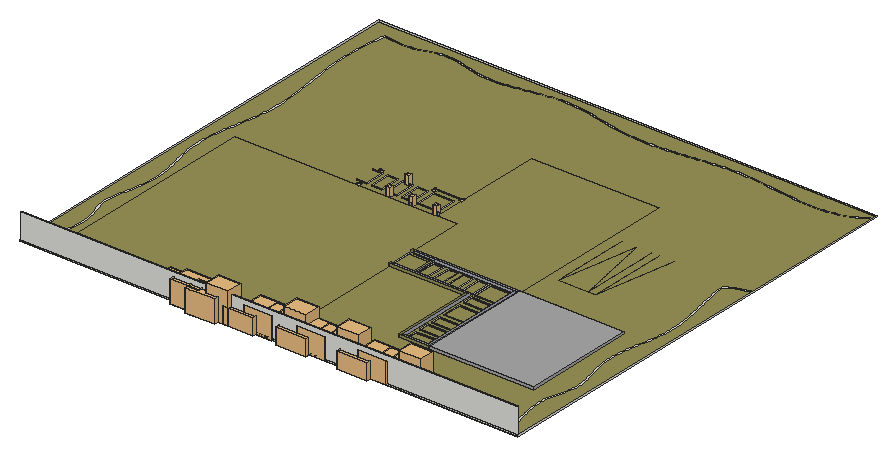
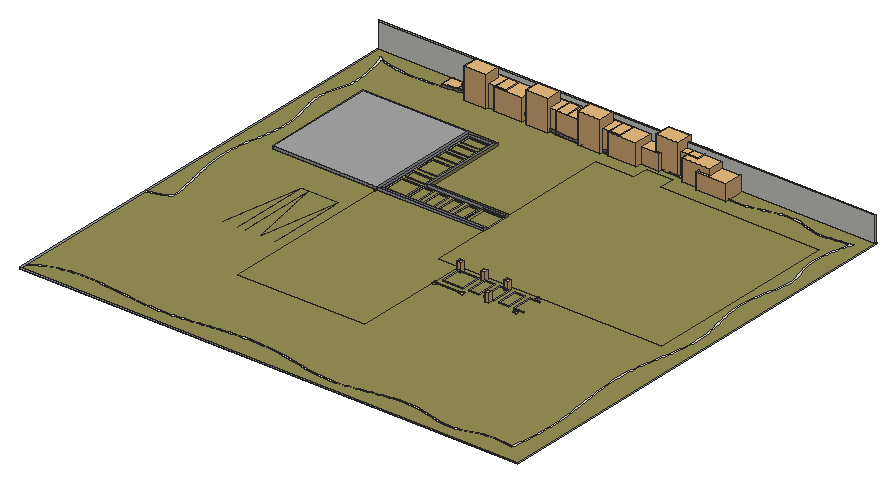
# SketchUp Ruby script. Lengths in inches.
U = 1.inch
M = Sketchup.active_model
def pt(a) = Geom::Point3d.new(a.map { |v| v * U })
def face(e, loops, mat)
  f = e.add_face(loops[0].map { |a| pt(a) })
  loops[1..].each { |l| e.add_face(l.map { |a| pt(a) }).erase! }
  f.material = f.back_material = mat if mat
  f
end
# faces: each face lists its corners as indices into pts; further lists are holes
def faces(e, pts, list, mat = nil) = list.each { |f| face(e, (f[0].is_a?(Array) ? f : [f]).map { |l| l.map { |i| pts[i] } }, mat) }
# xy, xz, yz: faces in a plane at the given z, y or x. An outline is a flat list of corners, or four numbers for a rectangle; further outlines are holes
def ring(l) = l.size == 4 ? [[l[0], l[1]], [l[2], l[1]], [l[2], l[3]], [l[0], l[3]]] : l.each_slice(2).to_a
def flat(e, list, mat, &to3) = list.each { |f| face(e, (f[0].is_a?(Array) ? f : [f]).map { |l| ring(l).map { |u, v| to3.(u, v) } }, mat) }
def xy(e, z, list, mat = nil) = flat(e, list, mat) { |x, y| [x, y, z] }
def xz(e, y, list, mat = nil) = flat(e, list, mat) { |x, z| [x, y, z] }
def yz(e, x, list, mat = nil) = flat(e, list, mat) { |y, z| [x, y, z] }
def lines(e, pts, list) = list.each { |a, b| e.add_line(pt(pts[a]), pt(pts[b])) }
# prism: a flat outline (further loops are holes) pulled along v
def prism(e, loops, v, mat = nil)
  f = face(e, loops, mat); d = Geom::Vector3d.new(v.map { |x| x * U })
  f.pushpull(f.normal.samedirection?(d) ? d.length : -d.length)
end
def box(e, o, s, mat = nil) = prism(e, [[o, [o[0] + s[0], o[1], o[2]], [o[0] + s[0], o[1] + s[1], o[2]], [o[0], o[1] + s[1], o[2]]]], [0, 0, s[2]], mat)
def at(x, y, z, deg = 0) = Geom::Transformation.translation(pt([x, y, z])) * Geom::Transformation.rotation(ORIGIN, Z_AXIS, deg.degrees)
def axes(o, x, y, z) = Geom::Transformation.new([*x, 0, *y, 0, *z, 0, *pt(o).to_a, 1])
def part(name) = M.definitions.add(name)
# library, detail: a bought-in or finely detailed component or shape, given as its bounding box
def library(name, o, s) = part(name).tap { |d| box(d.entities, o, s) }
def detail(e, o, s) = box(e.add_group.entities, o, s)
def put(e, d, t, mat = nil) = e.add_instance(d, t).tap { |i| i.material = mat if mat }
def group(e, t, mat = nil) = e.add_group.tap { |g| g.transformation = t; g.material = mat if mat }.entities
root = M.entities
M.materials.add("M03_Pewter_Shine").color = [168, 168, 168]
M.materials.add("Marble_01_1K").color = [230, 221, 211]
M.materials.add("Marble_20_1K").color = [172, 173, 182]
M.materials.add("Material__4").color = [36, 36, 36]
M.materials.add("Material__6").color = [79, 108, 5]
M.materials.add("Plaster_06_1K").color = [141, 135, 122]
M.materials.add("Soil_04_1K").color = [152, 146, 88]
M.materials.add("calathea lutea").color = [121, 145, 80]
c1 = library("light",[-4,-4,0],[8,8,0.01])
c2 = library("tt",[-12.4,-12.1,0],[24.8,24.2,0.01])
c3 = library("ew",[-14.92,-16.84,0],[29.84,33.68,0.01])
c4 = part("Group\#156")
g1 = group(c4.entities,at(8.61,38.85,0))
xy(g1,0,[[0,0,2.82,19.1,22.58,0],[22.58,0,2.82,19.1,22.58,19.1]],"calathea lutea")
p = [[2.82,19.1,0],[7.19,48.22,5.13],[10.77,48.22,5.13],[12.74,48.22,5.13],[22.58,48.22,5.13],[22.58,19.1,0]]
faces(g1,p,[[0,1,2,3,4,5]],"calathea lutea")
g2 = group(c4.entities,at(-0.77,-7.77,0))
p = [[14.8125,23.31,1.46],[21.35,23.31,0],[14.8125,0,1.46],[21.35,0,0],[27.89,0,1.46],[27.89,23.31,1.46],
  [8.27,46.62,2.92],[21.35,46.62,0],[34.4375,46.62,2.92],[4.47,23.31,6.43],[0,0,8.59],[33.76,0,4.28],
  [33.76,23.31,4.28]]
faces(g2,p,[[0,1,2],[3,2,1],[4,3,5],[1,5,3],[6,7,0],[1,0,7],[5,1,8],[7,8,1],
  [9,0,2,10],[11,4,5,12],[9,6,0],[12,5,8]],"calathea lutea")
c5 = part("Group\#150")
xy(c5.entities,0,[[0,0,0,33.87,27.21,33.87,19.71,0]],"calathea lutea")
c6 = part("Group\#157")
xy(c6.entities,1.04,[[21.13,33.87,21.13,57.59,32.375,57.59,27.12,33.87]],"calathea lutea")
xy(c6.entities,1.32,[[0.12,33.87,7.74,57.59]],"calathea lutea")
p = [[7.74,33.87,1.32],[11.8,57.59,0.61],[15.24,57.59,0],[15.24,33.87,0],[18.43,57.59,0.5625],[21.13,57.59,1.04],
  [21.13,33.87,1.04],[15.24,77.7,2.36],[21.13,77.7,3.4],[7.74,57.59,1.32],[7.74,77.7,3.69],[36.83,77.7,3.4],
  [32.375,57.59,1.04],[0.12,57.59,1.32],[0.12,77.7,3.69]]
faces(c6.entities,p,[[0,1,2,3],[3,2,4],[3,4,5,6],[7,2,1],[8,4,2,7],[0,9,1],[7,1,9,10],[8,5,4],
  [11,12,5,8],[10,9,13,14]],"calathea lutea")
put(c6.entities,c5,axes([0,-16.9375,0],[1,0,0],[0,1.5,0],[0,0,1]))
c7 = part("Group\#155")
g3 = group(c7.entities,at(0,-17.3,0))
xy(g3,0,[[0,0,28.07,51.9]],"calathea lutea")
g4 = group(c7.entities,at(0.9,34.6,0))
xy(g4,0,[[13.14,0,13.14,26.22,16.85,26.22],[13.14,0,16.85,26.22,20.16,26.22,20.16,0]],"calathea lutea")
p = [[6.36,0,1.82],[9.95,26.22,0.86],[13.14,26.22,0],[13.14,0,0],[20.16,0,0],[20.16,26.22,0],
  [27.07,26.22,1.22],[27.07,0,1.22],[13.14,49.5625,5.91],[20.16,49.5625,5.91],[16.85,26.22,0],[27.07,49.5625,7.125],
  [6.36,26.22,1.82],[6.36,49.5625,7.72],[0,0,4.78],[0,26.22,4.78],[0,49.5625,10.6875]]
faces(g4,p,[[0,1,2,3],[4,5,6,7],[8,2,1],[9,10,2,8],[9,5,10],[11,6,5,9],[0,12,1],[8,1,12,13],
  [14,15,12,0],[13,12,15,16]],"calathea lutea")
c8 = part("Group\#154")
put(c8.entities,c5,axes([0,-16.9375,0],[1,0,0],[0,1.5,0],[0,0,1]))
g5 = group(c8.entities,at(-0.23,33.4,-0.35))
p = [[15.12,39.14,-19.87],[15.12,20.54,-11.86],[11.68,20.84,-11.33],[21.02,39.66,-18.97],[18.3125,20.82,-11.37],[7.62,21.2,-10.71],
  [7.62,39.8,-18.72],[21.02,21.06,-10.96],[36.72,39.66,-18.97],[32.26,21.06,-10.96],[0,21.2,-10.71],[0,39.8,-18.72],
  [7.62,0.66,1.15],[15.12,0,0],[21.02,0.52,0.9],[27.01,0.52,0.9],[0,0.66,1.15]]
faces(g5,p,[[0,1,2],[3,4,1,0],[0,2,5,6],[3,7,4],[8,9,7,3],[6,5,10,11],[12,2,1,13],[13,1,4],
  [13,4,7,14],[12,5,2],[14,7,9,15],[16,10,5,12]],"calathea lutea")
c9 = part("Foliage cluster")
put(c9.entities,c4,axes([37.24,8.07,75.17],[1,0,0],[0,0.45554,-0.89021],[0,0.89021,0.45554]))
put(c9.entities,c6,axes([69.44,65.48,16.68],[-0.53288,-0.84619,0],[0.14694,-0.09253,0.98481],[-0.83334,0.52478,0.17365]))
put(c9.entities,c7,axes([47.9375,70.43,17.04],[0.74664,-0.66523,0],[0.11552,0.12965,0.98481],[-0.65512,-0.7353,0.17365]))
put(c9.entities,c4,axes([76.19,10.66,75.17],[0.70711,0.70711,0],[-0.32212,0.32212,-0.89021],[-0.62948,0.62948,0.45554]))
put(c9.entities,c4,axes([101.91,40.03,75.17],[0,1,0],[-0.45554,0,-0.89021],[-0.89021,0,0.45554]))
put(c9.entities,c4,axes([99.32,78.99,75.17],[-0.70711,0.70711,0],[-0.32212,-0.32212,-0.89021],[-0.62948,-0.62948,0.45554]))
put(c9.entities,c7,axes([34.81,63.36,17.04],[0.99956,-0.02967,0],[0.00515,0.17357,0.98481],[-0.02922,-0.98437,0.17365]))
put(c9.entities,c7,axes([48,37.4,15.8],[-0.14436,0.98953,0],[-0.40248,-0.05871,0.91355],[0.90398,0.13188,0.40674]))
put(c9.entities,c6,axes([56.87,39.77,12.28],[-0.67695,0.4263,0],[-0.18016,-0.28609,0.72505],[0.38636,0.61353,0.33809]))
put(c9.entities,c6,axes([36.12,43.25,12.28],[0.18947,0.77724,0],[-0.32848,0.08007,0.72505],[0.70442,-0.17172,0.33809]))
put(c9.entities,c8,axes([35.1,54.93,11.375],[0.79719,0.06694,0],[-0.03636,0.43302,0.6717],[0.05621,-0.66934,0.43454]))
put(c9.entities,c6,axes([41.66,47.32,12.28],[0.45082,0.66088,0],[-0.2793,0.19053,0.72505],[0.59896,-0.40858,0.33809]))
put(c9.entities,c6,axes([47.89,59.4,12.28],[0.79719,0.06694,0],[-0.02829,0.33691,0.72505],[0.06067,-0.7225,0.33809]))
put(c9.entities,c8,axes([29.53,49.96,11.375],[0.65692,0.45657,0],[-0.248,0.35682,0.6717],[0.38335,-0.55156,0.43454]))
put(c9.entities,c8,axes([29.9,49.27,12.86],[0.34062,0.72386,0],[-0.22849,0.10752,0.7591],[0.68685,-0.32321,0.25252]))
put(c9.entities,c8,axes([36.33,48.82,8.99],[0.09232,0.62522,0],[-0.3396,0.05015,0.53064],[0.52495,-0.07752,0.34329]))
put(c9.entities,c8,axes([49.82,38.52,8.99],[-0.54622,0.31791,0],[-0.17268,-0.29669,0.53064],[0.26692,0.45862,0.34329]))
put(c9.entities,c8,axes([55.68,39.21,8.99],[-0.632,0.00221,0],[-0.0012,-0.34328,0.53064],[0.00185,0.53064,0.34329]))
c10 = library("Group\#28",[0,0,0],[86.94,78.77,46.4375])
c11 = library("Group\#14",[-978.71,-103.24,719.12],[90.2,76.4,68.29])
c12 = library("Group\#13",[-906.16,-138.28,686.8],[98.25,106.18,75.79])
c13 = library("Group\#202",[-3.47,-2.45,12.47],[53.14,54.93,75.51])
c14 = library("Group\#54",[0,0,0],[2062.46,2062.46,4833.66])
c15 = part("Landscape+Light")
put(c15.entities,c14,at(-2096.57,-1031.23,-3775.98))
c16 = library("t1",[-17.79,-17.21,0],[35.58,34.42,0.01])
c17 = part("Group\#44")
put(c17.entities,c9,axes([161.54,105.34,6.01],[0.19523,-0.19694,0],[0.19694,0.19523,0],[0,0,0.24957]))
put(c17.entities,c10,axes([0,37.34,0.92],[0.83,0,0],[0,0.83,0],[0,0,0.83]))
put(c17.entities,c11,axes([859.63,139.86,-568.1],[0.79,0,0],[0,0.79,0],[0,0,0.79]),"Material__4")
put(c17.entities,c12,axes([669.69,145.1,-472.48],[0.69,0,0],[0,0.69,0],[0,0,0.69]),"Material__6")
put(c17.entities,c13,at(132.78,74.93,-12.6))
xy(root,0,[[480.859,22.514,469.576,22.663,458.203,23.333,446.764,24.525,435.279,26.15,423.754,28.103,412.194,30.286,400.608,32.597,389.002,34.937,377.385,37.206,365.763,39.306,354.147,41.14,342.544,42.61,330.964,43.618,319.414,44.07,307.903,43.869,296.431,42.924,284.954,41.245,273.478,39.01,262.023,36.415,250.609,33.658,239.255,30.938,227.977,28.456,216.79,26.418,205.705,25.031,194.737,24.507,183.905,25.065,173.26,26.904,162.899,29.804,152.679,33.204,142.425,36.559,131.969,39.345,121.109,41.119,109.806,41.864,98.284,41.752,86.773,40.964,75.503,39.681,64.7,38.09,54.587,36.377,45.348,34.713,36.369,33.075,37.514,35.489,38.66,37.904,39.808,40.342,41.005,43.315,42.25,47.021,43.529,51.453,44.835,56.612,46.164,62.502,47.513,69.13,48.883,76.509,50.312,84.622,51.732,93.308,53.035,102.439,54.109,111.884,54.846,121.51,55.138,131.183,54.879,140.766,53.965,150.125,52.298,159.138,49.937,167.888,47.159,176.49,44.27,185.043,41.586,193.648,39.4375,202.41,38.14,211.376,37.733,220.458,38.089,229.635,39.079,238.896,40.576,248.232,42.459,257.636,44.605,267.101,46.895,276.617,49.21,286.176,51.434,295.765,53.449,305.374,55.14,314.99,56.393,324.601,57.112,334.213,57.309,343.854,57.039,353.523,56.36,363.215,55.325,372.925,53.993,382.649,52.42,392.381,50.664,402.117,48.783,411.85,46.833,421.576,44.873,431.291,42.962,440.991,41.158,450.67,39.521,460.325,38.109,469.951,36.982,479.546,36.201,489.105,35.799,498.606,35.753,508.044,36.031,517.421,36.604,526.741,37.439,536.006,38.507,545.221,39.776,554.389,41.216,563.513,42.797,572.596,44.486,581.644,46.256,590.658,48.074,599.642,49.912,608.601,51.739,617.537,53.524,626.455,55.239,635.357,56.852,644.248,58.336,653.13,59.659,662.006,60.793,670.882,61.708,679.759,62.385,688.651,62.836,697.561,63.075,706.489,63.117,715.435,62.976,724.398,62.669,733.377,62.209,742.37,61.613,751.377,60.895,760.397,60.07,769.428,59.153,778.469,58.159,787.52,57.104,796.579,56.004,805.645,54.872,814.718,53.725,823.796,52.578,832.878,51.446,841.963,50.344,851.051,49.287,860.139,48.292,869.229,47.373,878.317,46.547,887.404,45.828,896.488,45.232,905.569,44.774,914.645,44.47,923.716,44.336,932.78,44.388,941.837,44.633,950.881,45.057,959.917,45.639,968.957,46.358,978.013,47.193,987.098,48.123,996.223,49.126,1005.402,50.183,1014.646,51.273,1023.969,52.374,1033.383,53.47,1042.887,63.941,1041.194,74.718,1039.586,85.979,1038.273,97.499,1037.444,109.045,1037.281,120.387,1037.965,131.296,1039.672,141.787,1042.409,152.064,1045.749,162.297,1049.166,172.66,1052.115,183.306,1054.029,194.148,1054.654,205.125,1054.182,216.221,1052.832,227.421,1050.819,238.712,1048.35,250.08,1045.633,261.509,1042.869,272.98,1040.258,284.474,1038.001,295.969,1036.292,307.458,1035.315,318.985,1035.087,330.551,1035.517,342.148,1036.509,353.768,1037.967,365.402,1039.794,377.041,1041.891,388.677,1044.16,400.301,1046.503,411.905,1048.82,423.483,1051.01,435.027,1052.972,446.531,1054.607,457.988,1055.811,469.38,1056.492,480.682,1056.65,491.897,1056.336,503.03,1055.604,514.087,1054.507,525.073,1053.098,535.995,1051.428,546.859,1049.551,557.67,1047.517,568.436,1045.38,579.161,1043.19,589.853,1040.999,600.516,1038.859,611.158,1036.82,621.784,1034.934,632.4,1033.251,643.011,1031.822,653.624,1030.696,664.256,1029.907,674.915,1029.439,685.6,1029.266,696.309,1029.363,707.041,1029.703,717.794,1030.262,728.567,1031.013,739.357,1031.931,750.162,1032.99,760.981,1034.164,771.812,1035.426,782.653,1036.752,793.503,1038.115,804.36,1039.488,815.221,1040.846,826.086,1042.163,836.953,1043.412,847.819,1044.567,858.684,1045.601,869.546,1046.488,880.403,1047.202,891.253,1047.716,902.095,1048.004,912.927,1048.038,923.744,1047.798,934.548,1047.297,945.358,1046.573,956.196,1045.662,967.083,1044.598,978.04,1043.418,989.088,1042.158,1000.249,1040.852,1011.544,1039.536,1022.995,1038.246,1034.624,1037.016,1046.425,1035.892,1058.357,1034.938,1070.374,1034.219,1082.429,1033.8,1094.476,1033.748,1106.468,1034.125,1118.359,1034.996,1130.102,1036.427,1141.651,1038.479,1152.963,1041.215,1163.991,1044.698,1174.694,1048.99,1185.032,1054.156,1194.964,1060.26,1204.463,1067.348,1204.463,1063.517,1194.306,1056.225,1183.681,1050.02,1172.637,1044.829,1161.225,1040.58,1149.495,1037.198,1137.499,1034.61,1125.287,1032.743,1112.909,1031.522,1100.417,1030.875,1087.86,1030.727,1075.29,1031.006,1062.757,1031.637,1050.312,1032.548,1038.005,1033.665,1025.886,1034.914,1013.972,1036.238,1002.24,1037.598,990.666,1038.954,979.229,1040.266,967.904,1041.497,956.667,1042.606,945.496,1043.554,934.367,1044.303,923.256,1044.8125,912.14,1045.045,901.005,1044.985,889.852,1044.659,878.682,1044.096,867.497,1043.324,856.3,1042.372,845.091,1041.27,833.874,1040.047,822.65,1038.731,811.42,1037.351,800.187,1035.937,788.953,1034.517,777.719,1033.12,766.488,1031.776,755.261,1030.513,744.04,1029.36,732.827,1028.347,721.624,1027.501,710.434,1026.854,699.257,1026.432,688.096,1026.265,676.953,1026.383,665.829,1026.814,654.726,1027.587,643.647,1028.724,632.585,1030.192,621.535,1031.934,610.49,1033.893,599.443,1036.013,588.388,1038.236,577.317,1040.506,566.224,1042.765,555.102,1044.958,543.944,1047.026,532.744,1048.913,521.494,1050.5625,510.189,1051.917,498.821,1052.92,487.384,1053.514,475.871,1053.643,464.275,1053.249,452.59,1052.287,440.82,1050.812,428.974,1048.933,417.061,1046.761,405.089,1044.407,393.068,1041.981,381.005,1039.594,368.911,1037.355,356.794,1035.377,344.663,1033.769,332.526,1032.642,320.393,1032.106,308.272,1032.272,296.173,1033.248,284.108,1035.019,272.098,1037.379,260.165,1040.104,248.328,1042.971,236.611,1045.755,225.033,1048.235,213.615,1050.185,202.379,1051.383,191.346,1051.605,180.537,1050.629,169.95,1048.319,159.451,1045.08,148.858,1041.508,137.986,1038.203,126.654,1035.76,114.824,1034.505,102.716,1034.276,90.578,1034.864,78.657,1036.056,67.199,1037.643,56.085,1039.364,54.849,1028.711,53.616,1018.189,52.414,1007.782,51.273,997.471,50.221,987.24,49.288,977.071,48.504,966.946,47.898,956.847,47.499,946.758,47.335,936.66,47.41,926.547,47.705,916.418,48.196,906.275,48.863,896.12,49.684,885.955,50.637,875.779,51.7,865.596,52.851,855.406,54.07,845.21,55.334,835.011,56.621,824.81,57.91,814.607,59.179,804.405,60.407,794.205,61.571,784.008,62.65,773.816,63.623,763.63,64.467,753.452,65.16,743.283,65.682,733.124,66.011,722.977,66.124,712.844,66,702.725,65.618,692.622,64.955,682.537,63.992,672.471,62.745,662.421,61.255,652.383,59.565,642.351,57.718,632.321,55.756,622.287,53.722,612.244,51.658,602.187,49.608,592.112,47.613,582.012,45.717,571.884,43.961,561.722,42.389,551.521,41.044,541.275,39.967,530.981,39.202,520.632,38.79,510.224,38.776,499.752,39.2,489.21,40.096,478.595,41.416,467.91,43.077,457.161,44.997,446.356,47.093,435.5,49.282,424.601,51.481,413.664,53.608,402.697,55.579,391.707,57.313,380.699,58.725,369.681,59.734,358.659,60.257,347.64,60.21,336.63,59.511,325.636,58.126,314.667,56.185,303.736,53.855,292.861,51.305,282.055,48.701,271.336,46.211,260.719,44.002,250.22,42.242,239.854,41.098,229.638,40.737,219.587,41.327,209.717,43.02,200.04,45.663,190.492,48.819,180.939,52.038,171.244,54.874,161.268,56.888,150.881,57.922,140.1,58.119,129.101,57.636,118.071,56.633,107.192,55.267,96.652,53.696,86.635,52.077,77.325,50.523,68.896,48.995,61.397,47.487,54.813,46.001,49.129,44.536,44.328,43.092,40.394,41.666,37.135,51.57,38.889,61.787,40.655,72.801,42.341,84.391,43.746,96.317,44.665,108.34,44.894,120.222,44.229,131.723,42.467,142.713,39.607,153.328,36.152,163.746,32.683,174.144,29.778,184.696,27.998,195.475,27.511,206.466,28.115,217.648,29.594,229,31.732,240.502,34.312,252.134,37.117,263.875,39.933,275.705,42.541,287.603,44.727,299.55,46.273,311.525,47.01,323.519,46.981,335.523,46.292,347.528,45.052,359.526,43.367,371.508,41.344,383.465,39.09,395.39,36.713,407.273,34.318,419.105,32.013,430.88,29.905,442.586,28.101,454.218,26.708,465.764,25.831,477.225,25.508,488.605,25.69,499.912,26.321,511.151,27.347,522.329,28.712,533.453,30.362,544.53,32.24,555.565,34.293,566.566,36.465,577.539,38.702,588.49,40.947,599.426,43.146,610.353,45.243,621.279,47.185,632.209,48.915,643.151,50.379,654.11,51.521,665.091,52.307,676.093,52.757,687.114,52.898,698.153,52.758,709.208,52.366,720.276,51.749,731.356,50.936,742.447,49.955,753.545,48.833,764.65,47.599,775.759,46.281,786.872,44.907,797.985,43.504,809.097,42.102,820.206,40.727,831.31,39.409,842.408,38.174,853.498,37.052,864.577,36.07,875.645,35.256,886.698,34.639,897.736,34.246,908.756,34.105,919.757,34.244,930.747,34.665,941.748,35.332,952.781,36.207,963.871,37.252,975.039,38.43,986.309,39.702,997.702,41.032,1009.243,42.38,1020.952,43.709,1032.854,44.981,1044.954,46.15,1057.211,47.15,1069.575,47.908,1081.999,48.353,1094.433,48.415,1106.827,48.023,1119.133,47.104,1131.302,45.588,1143.285,43.404,1155.033,40.481,1166.497,36.747,1177.627,32.131,1176.661,34.304,1175.695,36.527,1174.719,39.093,1173.734,42.055,1172.739,45.418,1171.734,49.186,1170.719,53.365,1169.695,57.96,1168.661,62.975,1167.617,68.415,1166.557,74.284,1165.459,80.555,1164.367,87.17,1163.328,94.072,1162.393,101.204,1161.61,108.508,1161.028,115.926,1160.696,123.401,1160.663,130.876,1160.979,138.293,1161.693,145.594,1162.854,152.722,1164.468,159.642,1166.419,166.384,1168.568,172.991,1170.775,179.506,1172.9,185.972,1174.806,192.43,1176.351,198.924,1177.405,205.495,1177.944,212.156,1178.02,218.902,1177.683,225.73,1176.987,232.633,1175.982,239.607,1174.722,246.647,1173.258,253.748,1171.641,260.906,1169.925,268.115,1168.162,275.37,1166.402,282.667,1164.699,290,1163.104,297.365,1161.669,304.757,1160.447,312.17,1159.489,319.601,1158.845,327.044,1158.519,334.496,1158.486,341.954,1158.72,349.418,1159.197,356.884,1159.889,364.351,1160.772,371.816,1161.82,379.278,1163.007,386.735,1164.306,394.184,1165.693,401.623,1167.142,409.051,1168.627,416.465,1170.122,423.863,1171.601,431.244,1173.039,438.604,1174.41,445.943,1175.689,453.258,1176.848,460.546,1177.864,467.806,1178.71,475.037,1179.36,482.234,1179.793,489.398,1180.012,496.53,1180.03,503.631,1179.862,510.703,1179.519,517.75,1179.016,524.773,1178.365,531.775,1177.58,538.758,1176.674,545.723,1175.661,552.674,1174.552,559.613,1173.363,566.542,1172.106,573.462,1170.794,580.377,1169.441,587.289,1168.059,594.2,1166.663,601.112,1165.264,608.027,1163.878,614.947,1162.516,621.876,1161.192,628.815,1159.92,635.766,1158.712,642.732,1157.581,649.715,1156.542,656.717,1155.607,663.741,1154.79,670.788,1154.104,677.862,1154.572,684.97,1160.145,692.147,1175.308,699.425,1204.463,706.821,1204.463,703.683,1176.673,696.07,1162.475,688.712,1157.456,681.529,1157.204,674.442,1157.945,667.378,1158.824,660.316,1159.828,653.253,1160.942,646.187,1162.151,639.118,1163.439,632.043,1164.792,624.96,1166.195,617.869,1167.634,610.766,1169.092,603.651,1170.555,596.522,1172.007,589.376,1173.433,582.212,1174.819,575.029,1176.148,567.823,1177.405,560.595,1178.576,553.341,1179.645,546.06,1180.596,538.751,1181.414,531.411,1182.084,524.038,1182.589,516.632,1182.914,509.189,1183.044,501.71,1182.963,494.191,1182.656,486.633,1182.108,479.036,1181.329,471.412,1180.347,463.768,1179.195,456.103,1177.901,448.421,1176.496,440.724,1175.009,433.013,1173.47,425.29,1171.908,417.557,1170.353,409.818,1168.835,402.073,1167.382,394.326,1166.023,386.58,1164.788,378.836,1163.705,371.097,1162.803,363.366,1162.11,355.645,1161.656,347.937,1161.469,340.244,1161.575,332.569,1162.005,324.913,1162.781,317.269,1163.879,309.619,1165.243,301.966,1166.816,294.318,1168.539,286.68,1170.354,279.059,1172.201,271.46,1174.022,263.888,1175.758,256.349,1177.347,248.847,1178.729,241.385,1179.842,233.968,1180.624,226.599,1181.012,219.283,1180.942,212.025,1180.346,204.83,1179.166,197.72,1177.455,190.748,1175.383,183.882,1173.117,177.07,1170.819,170.259,1168.646,163.4,1166.75,156.442,1165.28,149.333,1164.302,141.997,1163.772,134.471,1163.641,126.824,1163.855,119.127,1164.362,111.445,1165.106,103.848,1166.033,96.404,1167.089,89.177,1168.217,82.236,1169.362,75.643,1170.472,69.476,1171.556,63.797,1172.628,58.59,1173.687,53.849,1174.731,49.573,1175.76,45.758,1176.771,42.402,1177.76,39.506,1178.718,37.074,1179.638,35.072,1180.549,33.15,1181.461,31.229,1182.372,29.308,1183.284,27.387,1183.794,26.3125,1184.195,25.466,1173.842,30.55,1163.128,34.769,1152.093,38.186,1140.779,40.863,1129.231,42.863,1117.493,44.247,1105.612,45.08,1093.632,45.424,1081.602,45.344,1069.567,44.904,1057.573,44.168,1045.666,43.202,1033.892,42.071,1022.293,40.839,1010.869,39.548,999.6,38.234,988.463,36.932,977.4375,35.677,966.502,34.504,955.635,33.449,944.815,32.547,934.022,31.835,923.235,31.347,912.434,31.119,901.617,31.166,890.792,31.463,879.958,31.985,869.117,32.705,858.272,33.598,847.424,34.635,836.574,35.792,825.724,37.042,814.876,38.358,804.031,39.715,793.192,41.086,782.359,42.446,771.534,43.769,760.72,45.028,749.918,46.197,739.129,47.252,728.356,48.165,717.601,48.912,706.864,49.466,696.149,49.802,685.457,49.895,674.789,49.719,664.146,49.248,653.531,48.457,642.934,47.331,632.339,45.902,621.739,44.22,611.13,42.336,600.504,40.301,589.857,38.164,579.182,35.976,568.473,33.789,557.724,31.655,546.929,29.624,536.083,27.748,525.178,26.079,514.209,24.668,503.17,23.569,492.055,22.833],[811.725,356.108,859.725,356.125]])
xy(root,0,[[460.425,50.78,522.398,50.78,522.398,88.78,613.506,88.78,613.506,562.78,566.192,562.78,566.192,565.82,561.692,565.82,561.692,562.78,76.506,562.78,76.506,88.78,460.425,88.78],[[797.8125,154.932,797.8125,356.108,613.506,356.108,613.506,368.125,661.506,368.125,661.506,415.985,613.506,415.985,613.506,428.082,870.828,428.082,870.828,154.932],[803.8125,160.932,864.828,160.932,864.828,422.082,619.506,422.082,619.506,421.985,667.506,421.985,667.506,362.125,619.506,362.125,619.506,362.108,803.8125,362.108]],[[803.8125,160.932,864.828,160.932,864.828,422.082,619.506,422.082,619.506,421.985,667.506,421.985,667.506,362.125,619.506,362.125,619.506,362.108,803.8125,362.108],[811.725,368.125,859.725,415.985],[811.725,272.266,859.725,320.125],[673.506,368.125,697.506,416.125],[709.506,368.125,733.506,416.125],[745.506,368.125,769.506,416.125],[781.506,368.125,805.506,416.125],[811.725,164.125,859.725,188.125],[811.725,200.125,859.725,224.125],[811.725,236.125,859.725,260.125],[811.725,332.125,859.725,356.108]],[613.506,428.082,870.828,428.082,870.828,846.156,566.192,846.156,566.192,562.78,613.506,562.78]],"Soil_04_1K")
xz(root,0.952,[[8.463,0,1208.463,60]])
xz(root,4.952,[[12.463,0,1204.463,60]])
xz(root,154.932,[[797.8125,0,870.828,6]],"Soil_04_1K")
xz(root,160.932,[[803.8125,0,864.828,6]],"Marble_20_1K")
xz(root,164.125,[[811.725,0,859.725,2]],"Marble_01_1K")
xz(root,188.125,[[811.725,0,859.725,2]],"Marble_01_1K")
xz(root,200.125,[[811.725,0,859.725,2]],"Marble_01_1K")
xz(root,224.125,[[811.725,0,859.725,2]],"Marble_01_1K")
xz(root,236.125,[[811.725,0,859.725,2]],"Marble_01_1K")
xz(root,260.125,[[811.725,0,859.725,2]],"Marble_01_1K")
xz(root,272.266,[[811.725,0,859.725,2]],"Marble_01_1K")
xz(root,320.125,[[811.725,0,859.725,2]],"Marble_01_1K")
xz(root,332.125,[[811.725,0,859.725,2]],"Marble_01_1K")
xz(root,356.108,[[811.725,0,859.725,2]],"Marble_01_1K")
xz(root,356.108,[[613.506,0,797.8125,6]],"Soil_04_1K")
xz(root,362.108,[[619.506,0,803.8125,6]],"Marble_20_1K")
xz(root,362.125,[[619.506,0,667.506,2]],"Soil_04_1K")
xz(root,368.125,[[673.506,0,697.506,2],[709.506,0,733.506,2],[745.506,0,769.506,2],[781.506,0,805.506,2],[811.725,0,859.725,2]],"Marble_01_1K")
xz(root,415.985,[[811.725,0,859.725,2]])
xz(root,416.125,[[673.506,0,697.506,2],[709.506,0,733.506,2],[745.506,0,769.506,2],[781.506,0,805.506,2]])
xz(root,421.985,[[619.506,0,667.506,2]],"Soil_04_1K")
xz(root,422.082,[[619.506,0,864.828,6]],"Marble_20_1K")
xz(root,428.082,[[613.506,0,870.828,6]],"Marble_20_1K")
xz(root,565.82,[[561.692,0,566.192,6]],"Marble_20_1K")
xz(root,576.64,[[360.076,0,384.076,2],[396.076,0,420.076,2],[432.076,0,456.076,2],[468.076,0,492.076,2]],"Marble_01_1K")
xz(root,576.78,[[506.431,0,554.431,2]],"Marble_01_1K")
xz(root,624.64,[[360.076,0,384.076,2],[396.076,0,420.076,2],[432.076,0,456.076,2],[468.076,0,492.076,2],[506.431,0,554.431,2]],"Marble_01_1K")
xz(root,640.64,[[506.431,0,554.431,2]],"Marble_01_1K")
yz(root,384.076,[[576.64,0,624.64,2]],"Marble_01_1K")
yz(root,396.076,[[576.64,0,624.64,2]],"Marble_01_1K")
yz(root,420.076,[[576.64,0,624.64,2]],"Marble_01_1K")
yz(root,432.076,[[576.64,0,624.64,2]],"Marble_01_1K")
yz(root,456.076,[[576.64,0,624.64,2]],"Marble_01_1K")
yz(root,468.076,[[576.64,0,624.64,2]],"Marble_01_1K")
yz(root,492.076,[[576.64,0,624.64,2]],"Marble_01_1K")
yz(root,498.692,[[562.78,0,567.28,6]],"Marble_20_1K")
yz(root,506.431,[[576.78,0,624.64,2]],"Marble_01_1K")
yz(root,554.431,[[576.78,0,624.64,2]],"Marble_01_1K")
yz(root,561.692,[[565.82,0,567.28,6]],"Marble_20_1K")
yz(root,613.506,[[368.125,0,415.985,2]])
yz(root,613.506,[[356.108,0,356.108,6,362.108,6,362.108,2,368.125,2,368.125,0],[415.985,0,415.985,2,422.082,2,422.082,6,428.082,6,428.082,0]],"Soil_04_1K")
yz(root,619.506,[[362.108,0,362.125,2],[421.985,0,422.082,2]],"Soil_04_1K")
yz(root,667.506,[[362.125,0,421.985,2]],"Marble_20_1K")
yz(root,673.506,[[368.125,0,416.125,2]])
yz(root,697.506,[[368.125,0,416.125,2]],"Marble_01_1K")
yz(root,709.506,[[368.125,0,416.125,2]],"Marble_01_1K")
yz(root,733.506,[[368.125,0,416.125,2]],"Marble_01_1K")
yz(root,745.506,[[368.125,0,416.125,2]],"Marble_01_1K")
yz(root,769.506,[[368.125,0,416.125,2]],"Marble_01_1K")
yz(root,781.506,[[368.125,0,416.125,2]],"Marble_01_1K")
yz(root,797.8125,[[154.932,0,356.108,6]],"Soil_04_1K")
yz(root,803.8125,[[160.932,0,362.108,6]],"Marble_20_1K")
yz(root,805.506,[[368.125,0,416.125,2]],"Marble_01_1K")
yz(root,811.725,[[164.125,0,188.125,2],[200.125,0,224.125,2],[236.125,0,260.125,2],[272.266,0,320.125,2],[332.125,0,356.108,2],
  [368.125,0,415.985,2]],"Marble_01_1K")
yz(root,859.725,[[164.125,0,188.125,2],[200.125,0,224.125,2],[236.125,0,260.125,2],[272.266,0,320.125,2],[332.125,0,356.108,2],
  [368.125,0,415.985,2]])
yz(root,864.828,[[160.932,0,422.082,6]],"Marble_20_1K")
yz(root,870.828,[[428.082,-24,437.082,0]])
yz(root,870.828,[[154.932,-24,428.082,6]],"Marble_20_1K")
p = [[469.576,22.663,0],[480.859,22.514,0],[480.859,22.514,6],[469.576,22.663,6],[492.055,22.833,0],[492.055,22.833,6],
  [458.203,23.333,0],[458.203,23.333,6],[503.17,23.569,0],[503.17,23.569,6],[446.764,24.525,0],[446.764,24.525,6],
  [514.209,24.668,0],[514.209,24.668,6],[435.279,26.15,0],[435.279,26.15,6],[525.178,26.079,0],[525.178,26.079,6],
  [477.225,25.508,0],[465.764,25.831,0],[465.764,25.831,6],[477.225,25.508,6],[488.605,25.69,0],[488.605,25.69,6],
  [499.912,26.321,0],[499.912,26.321,6],[454.218,26.708,0],[454.218,26.708,6],[423.754,28.103,0],[423.754,28.103,6],
  [536.083,27.748,0],[536.083,27.748,6],[511.151,27.347,0],[511.151,27.347,6],[442.586,28.101,0],[442.586,28.101,6],
  [522.329,28.712,0],[522.329,28.712,6],[546.929,29.624,0],[546.929,29.624,6],[412.194,30.286,0],[412.194,30.286,6],
  [430.88,29.905,0],[430.88,29.905,6],[533.453,30.362,0],[533.453,30.362,6],[557.724,31.655,0],[557.724,31.655,6],
  [419.105,32.013,0],[419.105,32.013,6],[400.608,32.597,0],[400.608,32.597,6],[544.53,32.24,0],[544.53,32.24,6],
  [901.617,31.166,0],[912.434,31.119,0],[912.434,31.119,6],[901.617,31.166,6],[923.235,31.347,0],[923.235,31.347,6],
  [890.792,31.463,0],[890.792,31.463,6],[934.022,31.835,0],[934.022,31.835,6],[879.958,31.985,0],[879.958,31.985,6],
  [568.473,33.789,0],[568.473,33.789,6],[944.815,32.547,0],[944.815,32.547,6],[407.273,34.318,0],[407.273,34.318,6],
  [869.117,32.705,0],[869.117,32.705,6],[555.565,34.293,0],[555.565,34.293,6],[955.635,33.449,0],[955.635,33.449,6],
  [389.002,34.937,0],[389.002,34.937,6],[858.272,33.598,0],[858.272,33.598,6],[966.502,34.504,0],[966.502,34.504,6],
  [847.424,34.635,0],[847.424,34.635,6],[579.182,35.976,0],[579.182,35.976,6],[908.756,34.105,0],[897.736,34.246,0],
  [897.736,34.246,6],[908.756,34.105,6],[919.757,34.244,0],[919.757,34.244,6],[886.698,34.639,0],[886.698,34.639,6],
  [930.747,34.665,0],[930.747,34.665,6],[395.39,36.713,0],[395.39,36.713,6],[566.566,36.465,0],[566.566,36.465,6],
  [977.4375,35.677,0],[977.4375,35.677,6],[836.574,35.792,0],[836.574,35.792,6],[875.645,35.256,0],[875.645,35.256,6],
  [941.748,35.332,0],[941.748,35.332,6],[377.385,37.206,0],[377.385,37.206,6],[864.577,36.07,0],[864.577,36.07,6],
  [952.781,36.207,0],[952.781,36.207,6],[988.463,36.932,0],[988.463,36.932,6],[825.724,37.042,0],[825.724,37.042,6],
  [589.857,38.164,0],[589.857,38.164,6],[853.498,37.052,0],[853.498,37.052,6],[963.871,37.252,0],[963.871,37.252,6],
  [577.539,38.702,0],[577.539,38.702,6],[383.465,39.09,0],[383.465,39.09,6],[999.6,38.234,0],[999.6,38.234,6],
  [814.876,38.358,0],[814.876,38.358,6],[842.408,38.174,0],[842.408,38.174,6],[365.763,39.306,0],[365.763,39.306,6],
  [975.039,38.43,0],[975.039,38.43,6],[600.504,40.301,0],[600.504,40.301,6],[831.31,39.409,0],[831.31,39.409,6],
  [1010.869,39.548,0],[1010.869,39.548,6],[804.031,39.715,0],[804.031,39.715,6],[986.309,39.702,0],[986.309,39.702,6],
  [588.49,40.947,0],[588.49,40.947,6],[371.508,41.344,0],[371.508,41.344,6],[820.206,40.727,0],[820.206,40.727,6],
  [793.192,41.086,0],[793.192,41.086,6],[997.702,41.032,0],[997.702,41.032,6],[611.13,42.336,0],[611.13,42.336,6],
  [809.097,42.102,0],[809.097,42.102,6],[599.426,43.146,0],[599.426,43.146,6],[1009.243,42.38,0],[1009.243,42.38,6],
  [782.359,42.446,0],[782.359,42.446,6],[359.526,43.367,0],[359.526,43.367,6],[797.985,43.504,0],[797.985,43.504,6],
  [621.739,44.22,0],[621.739,44.22,6],[771.534,43.769,0],[771.534,43.769,6],[1020.952,43.709,0],[1020.952,43.709,6],
  [610.353,45.243,0],[610.353,45.243,6],[786.872,44.907,0],[786.872,44.907,6],[760.72,45.028,0],[760.72,45.028,6],
  [632.339,45.902,0],[632.339,45.902,6],[775.759,46.281,0],[775.759,46.281,6],[749.918,46.197,0],[749.918,46.197,6],
  [621.279,47.185,0],[621.279,47.185,6],[642.934,47.331,0],[642.934,47.331,6],[739.129,47.252,0],[739.129,47.252,6],
  [764.65,47.599,0],[764.65,47.599,6],[632.209,48.915,0],[632.209,48.915,6],[653.531,48.457,0],[653.531,48.457,6],
  [728.356,48.165,0],[728.356,48.165,6],[753.545,48.833,0],[753.545,48.833,6],[717.601,48.912,0],[717.601,48.912,6],
  [664.146,49.248,0],[664.146,49.248,6],[742.447,49.955,0],[742.447,49.955,6],[643.151,50.379,0],[643.151,50.379,6],
  [706.864,49.466,0],[706.864,49.466,6],[674.789,49.719,0],[674.789,49.719,6],[696.149,49.802,0],[696.149,49.802,6],
  [685.457,49.895,0],[685.457,49.895,6],[731.356,50.936,0],[731.356,50.936,6],[654.11,51.521,0],[654.11,51.521,6],
  [720.276,51.749,0],[720.276,51.749,6],[665.091,52.307,0],[665.091,52.307,6],[709.208,52.366,0],[709.208,52.366,6],
  [676.093,52.757,0],[676.093,52.757,6],[698.153,52.758,0],[698.153,52.758,6],[687.114,52.898,0],[687.114,52.898,6],
  [971.258,187.619,0],[971.258,187.618,0],[957.71,187.619,0],[957.71,187.618,0],[966.312,331.06,0],[966.311,331.06,0],
  [967.826,704.823,0],[967.826,512.779,0],[985.675,512.779,0],[661.506,415.985,0],[661.506,415.985,2],[661.506,368.125,0],
  [661.506,368.125,2],[985.675,704.823,0],[1021.589,704.824,0],[971.258,154.932,0],[971.258,154.93,0],[949.538,309.77,0],
  [949.537,309.771,0],[895.783,512.779,0],[895.783,704.823,0],[931.697,704.824,0],[870.828,437.082,-24],[1152.763,437.082,-24],
  [1152.763,154.932,-24],[870.828,154.932,-24],[957.71,154.932,0],[957.71,154.93,0]]
faces(root,p,[[0,1,2,3],[1,4,5,2],[6,0,3,7],[4,8,9,5],[10,6,7,11],[8,12,13,9],[14,10,11,15],[12,16,17,13],
  [28,14,15,29],[16,30,31,17],[30,38,39,31],[40,28,29,41],[38,46,47,39],[50,40,41,51],[54,55,56,57],[55,58,59,56],
  [60,54,57,61],[58,62,63,59],[64,60,61,65],[46,66,67,47],[62,68,69,63],[72,64,65,73],[68,76,77,69],[78,50,51,79],
  [80,72,73,81],[76,82,83,77],[84,80,81,85],[66,86,87,67],[82,102,103,83],[104,84,85,105],[110,78,79,111],[102,116,117,103],
  [118,104,105,119],[86,120,121,87],[116,130,131,117],[132,118,119,133],[136,110,111,137],[120,140,141,121],[130,144,145,131],[146,132,133,147],
  [156,146,147,157],[140,160,161,141],[168,156,157,169],[160,174,175,161],[176,168,169,177],[184,176,177,185],[174,186,187,175],[190,184,185,191],
  [186,194,195,187],[196,190,191,197],[194,202,203,195],[204,196,197,205],[208,204,205,209],[202,210,211,203],[216,208,209,217],[210,218,219,211],
  [220,216,217,221],[218,222,223,219],[222,220,221,223]])
faces(root,p,[[18,19,20,21],[22,18,21,23],[24,22,23,25],[19,26,27,20],[32,24,25,33],[26,34,35,27],[36,32,33,37],[34,42,43,35],
  [44,36,37,45],[42,48,49,43],[52,44,45,53],[48,70,71,49],[74,52,53,75],[88,89,90,91],[92,88,91,93],[89,94,95,90],
  [96,92,93,97],[70,98,99,71],[100,74,75,101],[94,106,107,95],[108,96,97,109],[106,112,113,107],[114,108,109,115],[112,122,123,113],
  [124,114,115,125],[126,100,101,127],[98,128,129,99],[122,134,135,123],[138,124,125,139],[134,142,143,135],[148,138,139,149],[150,126,127,151],
  [128,152,153,129],[142,154,155,143],[158,148,149,159],[154,162,163,155],[164,150,151,165],[166,158,159,167],[152,170,171,153],[162,172,173,163],
  [178,166,167,179],[180,164,165,181],[172,182,183,173],[182,188,189,183],[192,180,181,193],[188,198,199,189],[200,192,193,201],[198,206,207,199],
  [206,212,213,207],[214,200,201,215],[212,224,225,213],[226,214,215,227],[224,228,229,225],[230,226,227,231],[228,232,233,229],[234,230,231,235],
  [232,236,237,233],[238,234,235,239],[236,238,239,237]],"Plaster_06_1K")
lines(root,p,[[240,241],[242,243],[244,245],[246,247],[247,248],[249,250],[251,252],[248,253],[248,254],[255,256],[257,258],[259,247],
  [260,259],[259,261],[262,263],[264,265],[261,247],[266,267]])
put(root,c1,at(372.08,566.89,0))
put(root,c1,at(372.08,632.3,0))
put(root,c2,axes([385.58,18.42,0],[0,-1,0],[-1,0,0],[0,0,1]))
put(root,c3,axes([422.02,20.08,0],[0,-1,0],[-1,0,0],[0,0,1]))
g6 = group(root,at(333.01,-21.13,-5.25))
put(g6,c9,axes([161.54,36.86,6.01],[0.19523,-0.13282,0],[0.19694,0.13166,0],[0,0,0.24957]))
put(g6,c10,axes([0,25.1875,0.92],[0.83,0,0],[0,0.55977,0],[0,0,0.83]))
put(g6,c11,axes([859.63,60.14,-568.1],[0.79,0,0],[0,0.53279,0],[0,0,0.79]),"Material__4")
put(g6,c12,axes([669.69,77.07,-472.48],[0.69,0,0],[0,0.46535,0],[0,0,0.69]),"Material__6")
put(g6,c13,axes([132.78,16.35,-12.6],[1,0,0],[0,0.67442,0],[0,0,1]))
put(root,c15,axes([437.42,571.62,13.79],[-0.0044,0,0],[0,-0.0044,0],[0,0,0.0044]))
put(root,c15,axes([437.42,629.125,13.79],[-0.0044,0,0],[0,-0.0044,0],[0,0,0.0044]))
put(root,c16,axes([466.26,17.9375,0],[0,-1,0],[-1,0,0],[0,0,1]))
put(root,c1,at(498.19,639.15,0,90))
put(root,c15,axes([498.8125,565.54,13.79],[0,-0.0044,0],[0.0044,0,0],[0,0,0.0044]))
put(root,c2,axes([507.92,18.42,0],[0,-1,0],[-1,0,0],[0,0,1]))
put(root,c3,axes([544.36,20.08,0],[0,-1,0],[-1,0,0],[0,0,1]))
put(root,c15,axes([556.32,565.54,13.79],[0,-0.0044,0],[0.0044,0,0],[0,0,0.0044]))
put(root,c1,at(561.9,639.15,0,90))
put(root,c16,axes([588.6,17.9375,0],[0,-1,0],[-1,0,0],[0,0,1]))
put(root,c17,axes([503.55,-33.03,-5.25],[1,0,0],[0,0.67442,0],[0,0,1]))
g7 = group(root,at(8.46,0.95,-3))
xy(g7,0,[[0,0,1200,1079.78]],"Soil_04_1K")
xz(g7,0,[[0,0,1200,3]])
xz(g7,1079.78,[[0,0,1200,3]])
yz(g7,0,[[0,0,1079.78,3]])
yz(g7,1200,[[0,0,1079.78,3]])
put(root,c2,axes([623.12,18.42,0],[0,-1,0],[-1,0,0],[0,0,1]))
put(root,c3,axes([659.55,20.08,0],[0,-1,0],[-1,0,0],[0,0,1]))
put(root,c16,axes([703.79,17.9375,0],[0,-1,0],[-1,0,0],[0,0,1]))
put(root,c17,axes([630.5,-33.03,-5.25],[1,0,0],[0,0.67442,0],[0,0,1]))
put(root,c2,axes([741.88,18.42,0],[0,-1,0],[-1,0,0],[0,0,1]))
put(root,c3,axes([778.32,20.08,0],[0,-1,0],[-1,0,0],[0,0,1]))
put(root,c16,axes([822.5625,17.9375,0],[0,-1,0],[-1,0,0],[0,0,1]))
put(root,c2,axes([859.96,18.42,0],[0,-1,0],[-1,0,0],[0,0,1]))
put(root,c17,axes([778.9,-33.03,-5.25],[1,0,0],[0,0.67442,0],[0,0,1]))
put(root,c3,axes([896.4,20.08,0],[0,-1,0],[-1,0,0],[0,0,1]))
put(root,c16,axes([940.64,17.9375,0],[0,-1,0],[-1,0,0],[0,0,1]))
put(root,c2,axes([975.16,18.42,0],[0,-1,0],[-1,0,0],[0,0,1]))
g8 = group(root,at(870.83,154.93,0))
box(g8,[0,0,0],[252,273.15,6],"M03_Pewter_Shine")
put(root,c3,axes([1011.6,20.08,0],[0,-1,0],[-1,0,0],[0,0,1]))
